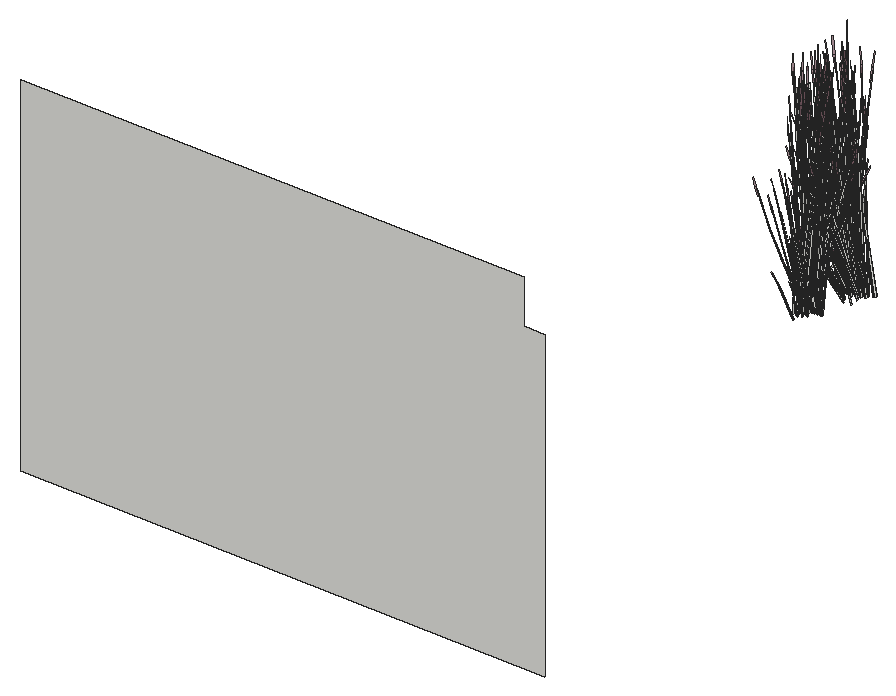
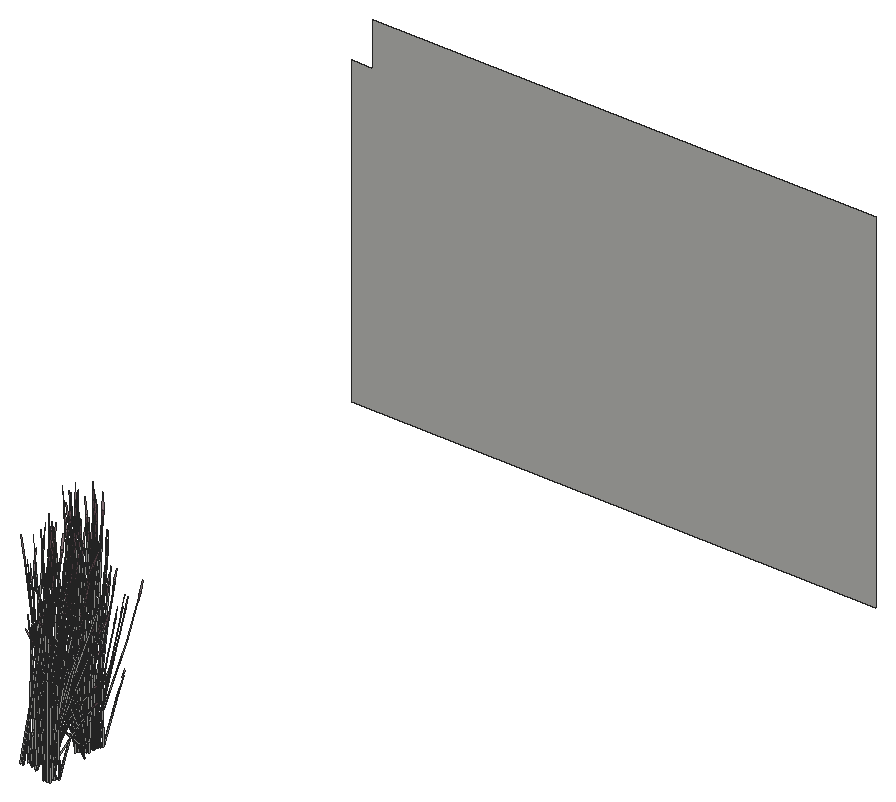
# SketchUp Ruby script. Lengths in inches.
U = 1.inch
M = Sketchup.active_model
def pt(a) = Geom::Point3d.new(a.map { |v| v * U })
def face(e, loops, mat)
  f = e.add_face(loops[0].map { |a| pt(a) })
  loops[1..].each { |l| e.add_face(l.map { |a| pt(a) }).erase! }
  f.material = f.back_material = mat if mat
  f
end
# faces: each face lists its corners as indices into pts; further lists are holes
def faces(e, pts, list, mat = nil) = list.each { |f| face(e, (f[0].is_a?(Array) ? f : [f]).map { |l| l.map { |i| pts[i] } }, mat) }
# xy, xz, yz: faces in a plane at the given z, y or x. An outline is a flat list of corners, or four numbers for a rectangle; further outlines are holes
def ring(l) = l.size == 4 ? [[l[0], l[1]], [l[2], l[1]], [l[2], l[3]], [l[0], l[3]]] : l.each_slice(2).to_a
def flat(e, list, mat, &to3) = list.each { |f| face(e, (f[0].is_a?(Array) ? f : [f]).map { |l| ring(l).map { |u, v| to3.(u, v) } }, mat) }
def xy(e, z, list, mat = nil) = flat(e, list, mat) { |x, y| [x, y, z] }
def xz(e, y, list, mat = nil) = flat(e, list, mat) { |x, z| [x, y, z] }
def yz(e, x, list, mat = nil) = flat(e, list, mat) { |y, z| [x, y, z] }
def lines(e, pts, list) = list.each { |a, b| e.add_line(pt(pts[a]), pt(pts[b])) }
# prism: a flat outline (further loops are holes) pulled along v
def prism(e, loops, v, mat = nil)
  f = face(e, loops, mat); d = Geom::Vector3d.new(v.map { |x| x * U })
  f.pushpull(f.normal.samedirection?(d) ? d.length : -d.length)
end
def box(e, o, s, mat = nil) = prism(e, [[o, [o[0] + s[0], o[1], o[2]], [o[0] + s[0], o[1] + s[1], o[2]], [o[0], o[1] + s[1], o[2]]]], [0, 0, s[2]], mat)
def at(x, y, z, deg = 0) = Geom::Transformation.translation(pt([x, y, z])) * Geom::Transformation.rotation(ORIGIN, Z_AXIS, deg.degrees)
def axes(o, x, y, z) = Geom::Transformation.new([*x, 0, *y, 0, *z, 0, *pt(o).to_a, 1])
def part(name) = M.definitions.add(name)
# library, detail: a bought-in or finely detailed component or shape, given as its bounding box
def library(name, o, s) = part(name).tap { |d| box(d.entities, o, s) }
def detail(e, o, s) = box(e.add_group.entities, o, s)
def put(e, d, t, mat = nil) = e.add_instance(d, t).tap { |i| i.material = mat if mat }
def group(e, t, mat = nil) = e.add_group.tap { |g| g.transformation = t; g.material = mat if mat }.entities
root = M.entities
M.materials.add("LightPink_Translucent").color = [144, 107, 117]
M.materials["LightPink_Translucent"].alpha = 0.75
c1 = part("blade")
p = [[2.15,0.21,22],[0,0.17,0],[0.09,0.45,0],[2.18,0.31,22],[2.29,0.31,22],[0.38,0.45,0],
  [2.48,0.24,33],[2.49,0.24,33],[2.48,0.22,33]]
faces(c1.entities,p,[[0,1,2,3],[4,5,2,3],[6,3,4,7],[8,0,3,6]])
c2 = part("seeds")
p = [[0.3,-0.1,1.38],[-0.01,-0.03,1.59],[-0.01,-0.03,0.03],[0.14,-0.07,-0.07],[0.29,-0.03,3],[0.15,0.01,3.11]]
faces(c2.entities,p,[[0,1,2,3],[1,0,4,5]],"LightPink_Translucent")
c3 = part("blade with seeds")
put(c3.entities,c1,at(0,0,0))
put(c3.entities,c2,axes([2.4,0.25,30.99],[1.5799,-0.05474,1.17369],[-0.12525,1.92788,0.29478],[-0.07173,-0.02425,1.56792]))
xz(root,279,[[198,0,342,0,342,84,336,84,336,96,198,96]])
put(root,c3,axes([289.94,432.61,2.59],[-0.25429,0.13207,1.43002],[-0.76157,-0.23115,-0.30754],[0.14117,-0.28747,0.61141]))
put(root,c3,axes([288.78,433.07,4.98],[-0.42698,-0.53052,-0.71045],[0.87893,-0.29566,0.08574],[-0.09984,-0.25633,1.00501]))
put(root,c3,axes([288.04,431.89,1.49],[-0.15005,0.02351,1.76342],[-0.82981,-0.26461,-0.26939],[0.01392,-0.22072,0.30037]))
put(root,c3,axes([290.55,433.59,4.98],[0.02328,-0.60353,-0.71045],[0.98022,0.04053,0.08574],[0.10344,-0.25568,1.00501]))
put(root,c3,axes([288.86,432.62,4.53],[0.2697,-0.50175,-0.35414],[0.78684,0.14635,0.4572],[-0.07215,-0.20201,0.87481]))
put(root,c3,axes([291.73,432.18,4.71],[-0.09085,0.04984,1.77383],[-0.89014,-0.16814,-0.16761],[-0.03222,-0.21748,0.31391]))
put(root,c3,axes([289,431.56,2.77],[0.11476,0.38047,1.1486],[-0.63664,-0.21072,0.84392],[0.06851,-0.19481,0.25299]))
put(root,c3,axes([290.36,433.39,4.68],[-0.64041,-0.4384,-0.51099],[0.67652,-0.38394,-0.3958],[0.09744,-0.22274,0.97773]))
put(root,c3,axes([288.95,432.74,4.73],[0.88151,0.17057,0.48003],[-0.30143,0.56078,0.3958],[-0.05297,-0.22053,0.9933]))
put(root,c3,axes([291.03,433.62,5.03],[-0.98321,-0.03233,-0.1216],[0.02687,-0.61208,-0.67495],[0.0683,-0.23574,1.02557]))
put(root,c3,axes([289.1875,432.69,4.73],[0.6592,-0.22175,0.0643],[0.32265,0.40436,0.50621],[-0.06366,-0.17825,0.77189]))
put(root,c3,axes([288.94,433.15,5.05],[-0.2697,0.50175,0.35414],[-0.78684,-0.14635,-0.4572],[-0.07215,-0.20201,0.87481]))
put(root,c3,axes([290.64,433.71,5.05],[-0.60531,0.34352,0.35414],[-0.573,-0.39225,-0.4572],[0.08718,-0.19929,0.87481]))
put(root,c3,axes([286.66,433.14,2.375],[-0.55932,-0.6538,0],[0.93577,-0.36461,-0.51607],[0.21313,-0.08304,1.63711]))
put(root,c3,axes([287.42,433.04,2.02],[0.83726,-0.32623,-0.49651],[0.50045,0.58498,0],[0.19069,-0.0743,1.57504]))
put(root,c3,axes([287.36,435.24,2.21],[0.43405,-0.58792,-0.44739],[0.90188,0.28295,0.21531],[0,-0.13553,1.43643]))
put(root,c3,axes([287.76,434.94,2.67],[-0.10425,-0.7445,-0.29095],[1.08575,-0.04502,-0.50002],[0.19119,-0.09917,1.59708]))
put(root,c3,axes([287.61,433.3,2.03],[0.83462,0.16144,-0.30978],[-0.21015,0.56852,0.30978],[0.16826,-0.06556,1.38974]))
put(root,c3,axes([287.9,435.53,2.43],[1.00799,0.31623,0.24065],[-0.48511,0.65709,0.50002],[0,-0.15147,1.60543]))
put(root,c3,axes([287.57,435.09,2.72],[-0.97146,0.04028,0.44739],[-0.08785,-0.66859,-0.21531],[0.17391,-0.06776,1.43643]))
put(root,c3,axes([287.54,435.33,2.36],[0.38895,0.72959,0.45755],[-1.11135,0.2537,0.17955],[0.01358,-0.13406,1.58856]))
put(root,c3,axes([287.34,435.9,2.72],[-0.43405,0.58792,0.44739],[-0.90188,-0.28295,-0.21531],[0,-0.13553,1.43643]))
put(root,c3,axes([288.9375,435.39,2.21],[0,-0.75495,0],[1.11865,0,0],[0,0,1.79456]))
put(root,c3,axes([290.29,433.65,2.48],[-0.83726,-0.32623,0.49651],[0.50045,-0.58498,0],[0.19069,0.0743,1.57504]))
put(root,c3,axes([288.41,434.91,2.36],[-0.74176,0.59212,0.45755],[-0.88124,-0.52269,0.17955],[0.17882,-0.05909,1.58856]))
put(root,c3,axes([289.22,435.97,2.3],[-0.83213,-0.56158,-0.06131],[0.83263,-0.56193,0],[-0.02906,-0.01961,1.75571]))
put(root,c3,axes([287.12,433.9375,2.47],[-0.25843,0.64844,0.17642],[-0.9457,-0.1835,0.35086],[0.16336,-0.00316,1.60407]))
put(root,c3,axes([289.09,434.66,2.62],[0.17258,-0.58229,0.1448],[0.84319,0.10108,-0.41347],[0.15345,0.05979,1.26744]))
put(root,c3,axes([288.73,434.8125,2.72],[-0.53742,-0.54764,0.44739],[0.81403,-0.38564,-0.21531],[0.17391,0.06776,1.43643]))
put(root,c3,axes([287.03,437.28,2.47],[0.96132,-0.17317,0.17642],[0.23737,0.64447,0.35086],[-0.08574,-0.0939,1.60407]))
put(root,c3,axes([289.7,435.56,2.21],[1.00089,0,0],[0,0.67548,0],[0,0,1.78407]))
put(root,c3,axes([289.98,433.97,2.47],[-0.96132,0.17317,0.17642],[-0.23737,-0.64447,0.35086],[0.08574,0.0939,1.60407]))
put(root,c3,axes([289.375,435.21,2.38],[-1.13071,-0.13747,0.49198],[0.23011,-0.77639,0.19306],[0.16524,0.07497,1.70813]))
put(root,c3,axes([288.47,437.13,2.2],[-0.29189,-0.56252,0],[0.83351,-0.19699,0],[0,0,1.54371]))
put(root,c3,axes([289.5625,437.05,2.18],[0.93921,-0.22138,-0.19198],[0.33003,0.6377,0.00008],[0.10367,-0.02447,1.73897]))
put(root,c3,axes([289.89,437.32,2.47],[0.25843,-0.64844,0.17642],[0.9457,0.1835,0.35086],[-0.16336,0.00316,1.60407]))
put(root,c3,axes([289.67,435.85,2.21],[0.62448,0.42144,0],[-0.62448,0.42144,0],[0,0,1.69266]))
put(root,c3,axes([291.37,435.66,2.47],[-0.70288,-0.47526,0.17642],[0.70832,-0.46097,0.35086],[-0.07763,0.09706,1.60407]))
put(root,c3,axes([288.27,437.39,2.2],[-0.90188,-0.29293,0],[0.43405,-0.60866,0],[0,0,1.62707]))
put(root,c3,axes([289.67,435.36,2.72],[0.43405,-0.58792,0.44739],[0.90188,0.28295,-0.21531],[0,0.13553,1.43643]))
put(root,c3,axes([289.5,435.69,2.29],[0,0.75458,-0.05637],[-1.11865,0,0],[0,0.02371,1.79368]))
put(root,c3,axes([291.94,435.68,2.48],[0,-0.65246,0.49651],[1.00089,0,0],[0,0.1486,1.57504]))
put(root,c3,axes([289.4375,436.17,2.72],[0.97146,-0.04028,0.44739],[0.08785,0.66859,-0.21531],[-0.17391,0.06776,1.43643]))
put(root,c3,axes([290.04,435.49,2.62],[0.83351,-0.19028,0.1448],[0.29189,0.54335,-0.41347],[0,0.11958,1.26744]))
put(root,c3,axes([289.29,437.4,2.2],[0.90188,0.29293,0],[-0.43405,0.60866,0],[0,0,1.74954]))
put(root,c3,axes([289.45,436.46,2.62],[0.66093,0.39201,0.1448],[-0.5513,0.44227,-0.41347],[-0.15345,0.05979,1.26744]))
put(root,c3,axes([290.16,437.67,2.48],[0.83726,-0.32623,0.49651],[0.50045,0.58498,0],[-0.19069,0.0743,1.57504]))
put(root,c3,axes([288.96,437.15,2.29],[0.38895,0.74956,-0.06012],[-1.11135,0.26265,0],[0.01358,0.02618,1.72173]))
put(root,c3,axes([292.18,436.17,2.2],[-1.1181,-0.00522,-0.04976],[0,-0.72922,0.49943],[-0.03514,0.166,1.58352]))
put(root,c3,axes([289.76,435.53,2.67],[1.00749,0.31132,-0.29095],[-0.48511,0.65709,-0.50002],[0.03166,0.16133,1.59708]))
put(root,c3,axes([292.51,444.75,3.875],[0.2045,0.20949,1.71376],[-0.94495,0.17636,0.13857],[-0.21357,-0.32887,0.73262]))
put(root,c3,axes([291.94,436.27,2.03],[-0.62448,0.40708,-0.30978],[-0.62448,-0.40708,0.30978],[0,0.13112,1.38974]))
put(root,c3,axes([289.65,436.02,2.21],[-0.43405,0.58792,-0.44739],[-0.90188,-0.28295,0.21531],[0,0.13553,1.43643]))
put(root,c3,axes([294.07,443.36,4.72],[-0.13683,-0.09148,1.74944],[-0.91315,0.058,-0.27667],[-0.14574,-0.2188,0.14031]))
put(root,c3,axes([295.02,444.9,4.98],[-0.42698,-0.53052,-0.71045],[0.87893,-0.29566,0.08574],[-0.09984,-0.25633,1.00501]))
put(root,c3,axes([292.25,444.19,2.59],[-0.05417,0.21344,1.43002],[-0.79196,0.17867,-0.30754],[-0.18512,-0.27588,0.61141]))
put(root,c3,axes([289.41,437.9,5.05],[-0.13817,-0.52554,0.35414],[0.78985,-0.13877,-0.4572],[0.21215,0.1506,0.87481]))
put(root,c3,axes([289.67,437.71,2.33],[1.11998,0.21207,0.30756],[-0.2802,0.75803,-0.36492],[-0.18537,0.09487,1.64885]))
put(root,c3,axes([292.375,436.29,2.02],[0,0.65246,-0.49651],[-1.00089,0,0],[0,0.1486,1.57504]))
put(root,c3,axes([294.7,444.8,4.68],[-0.87941,-0.16356,-0.51099],[0.30143,-0.56078,-0.3958],[-0.08064,-0.22578,0.97773]))
put(root,c3,axes([293.13,443.06,4.71],[-0.01669,0.07821,1.77383],[-0.82314,0.28383,-0.16761],[-0.24223,-0.14508,0.31391]))
put(root,c3,axes([290.35,438.12,2.375],[0.55932,0.6538,0],[-0.93577,0.36461,-0.51607],[-0.21313,0.08304,1.63711]))
put(root,c3,axes([290.16,436.2,2.09],[0.32803,0.59738,-0.69212],[-0.94492,0.21515,-0.18165],[0.03626,0.20229,1.52773]))
put(root,c3,axes([292.95,444.45,5.09],[0.99656,-0.1677,0.53763],[0.17295,0.65785,0.4433],[-0.23438,-0.19388,1.11249]))
put(root,c3,axes([287.52,437.99,5.05],[0.2697,-0.50175,0.35414],[0.78684,0.14635,-0.4572],[0.07215,0.20201,0.87481]))
put(root,c3,axes([295.46,444.77,5.03],[-0.87543,0.30377,-0.1216],[-0.4302,-0.53915,-0.67495],[-0.1155,-0.2272,1.02557]))
put(root,c3,axes([291.97,443.85,2.77],[0.46666,0.22709,1.1486],[-0.67962,0.13651,0.84392],[-0.14541,-0.17452,0.25299]))
put(root,c3,axes([293.1,445.05,4.98],[-0.76283,-0.31537,-0.71045],[0.54213,-0.55263,0.08574],[-0.27638,-0.1883,1.00501]))
put(root,c3,axes([292.84,444.64,4.53],[-0.13817,-0.52554,-0.35414],[0.78985,-0.13877,0.4572],[-0.21215,-0.1506,0.87481]))
put(root,c3,axes([289.53,438.38,4.73],[-0.4066,0.41448,0.0643],[-0.57901,-0.24131,0.50621],[0.18719,0.13288,0.77189]))
put(root,c3,axes([288.57,439.78,5.65],[0.61821,-0.37431,-0.06488],[0.56645,0.40995,-0.29416],[0.03988,0.11616,0.97024]))
put(root,c3,axes([289.7,438.27,4.73],[-0.88979,0.14973,0.48003],[-0.15442,-0.58737,0.3958],[0.20926,0.17311,0.9933]))
put(root,c3,axes([293.18,444.59,4.73],[0.4066,-0.41448,0.0643],[0.57901,0.24131,0.50621],[-0.18719,-0.13288,0.77189]))
put(root,c3,axes([291.6,444.53,1.49],[-0.08666,0.08595,1.76342],[-0.87574,0.18531,-0.26939],[-0.21156,-0.16858,0.30037]))
put(root,c3,axes([293.05,446.89,2.1],[-0.36739,-0.66907,-0.69835],[1.05831,-0.24096,-0.18329],[-0.04061,-0.22656,1.54149]))
put(root,c3,axes([287.27,438.44,4.73],[-0.6592,0.22175,0.0643],[-0.32265,-0.40436,0.50621],[0.06366,0.17825,0.77189]))
put(root,c3,axes([287.25,438.2,5.03],[0.87543,-0.30377,-0.1216],[0.4302,0.53915,-0.67495],[0.1155,0.2272,1.02557]))
put(root,c3,axes([287.51,438.4,5.0625],[-0.88151,-0.17057,0.53283],[0.30143,-0.56078,0.43934],[0.05297,0.22053,1.10256]))
put(root,c3,axes([292.74,445.07,4.68],[-0.88277,0.1551,-0.51099],[-0.15442,-0.58737,-0.3958],[-0.23711,-0.16832,0.97773]))
put(root,c3,axes([293.36,444.54,5.43],[-0.59706,0.6255,-0.13619],[-0.86465,-0.36036,-0.75594],[-0.30056,-0.17672,1.14864]))
put(root,c3,axes([287.41,438.32,1.49],[0.14478,-0.0355,1.76342],[0.8709,0.19542,-0.26939],[0.02547,0.22025,0.30037]))
put(root,c3,axes([294.13,444.18,2.13],[-0.61821,0.37431,-0.03893],[-0.56645,-0.40995,-0.17649],[-0.03988,-0.11616,0.58215]))
put(root,c3,axes([288,438.17,4.68],[0.87941,0.16356,-0.51099],[-0.30143,0.56078,-0.3958],[0.08064,0.22578,0.97773]))
put(root,c3,axes([288.5,437.02,3.875],[-0.2045,-0.20949,1.71376],[0.94495,-0.17636,0.13857],[0.21357,0.32887,0.73262]))
put(root,c3,axes([287.6,438.52,4.53],[-0.2697,0.50175,-0.35414],[-0.78684,-0.14635,0.4572],[0.07215,0.20201,0.87481]))
put(root,c3,axes([294.93,448.62,3.33],[0.77308,0.2631,1.51261],[-0.75736,0.56681,0.59816],[-0.33924,-0.33594,1.26806]))
put(root,c3,axes([293.3,445.0625,5.05],[0.13817,0.52554,0.35414],[-0.78985,0.13877,-0.4572],[-0.21215,-0.1506,0.87481]))
put(root,c3,axes([290.88,446.8,2.02],[0,-0.65246,-0.49651],[1.00089,0,0],[0,-0.1486,1.57504]))
put(root,c3,axes([287.68,438.07,4.98],[0.42698,0.53052,-0.71045],[-0.87893,0.29566,0.08574],[0.09984,0.25633,1.00501]))
put(root,c3,axes([291.27,445.4,4.73],[0.04505,-0.49615,0.0643],[0.68022,0.0136,0.50621],[-0.26056,-0.05192,0.77189]))
put(root,c3,axes([287.05,439.41,4.72],[0.1134,0.10507,1.74944],[0.91515,0.04128,-0.27667],[0.09203,0.23172,0.14031]))
put(root,c3,axes([291.3125,446.82,2.03],[0.62448,-0.40708,-0.30978],[0.62448,0.40708,0.30978],[0,-0.13112,1.38974]))
put(root,c3,axes([291.06,444.86,2.13],[-0.25807,0.53277,-0.03893],[-0.79428,-0.16389,-0.17649],[-0.1206,-0.08714,0.58215]))
put(root,c3,axes([293.5,447.56,2.67],[-1.00749,-0.31132,-0.29095],[0.48511,-0.65709,-0.50002],[-0.03166,-0.16133,1.59708]))
put(root,c3,axes([290.63,447.3,2.375],[-1.11865,0,0],[0,-0.72922,-0.51607],[0,-0.16609,1.63711]))
put(root,c3,axes([288.49,449.68,2.59],[-0.25429,0.13207,1.43002],[-0.76157,-0.23115,-0.30754],[0.14117,-0.28747,0.61141]))
put(root,c3,axes([286.6,448.96,1.49],[-0.15005,0.02351,1.76342],[-0.82981,-0.26461,-0.26939],[0.01392,-0.22072,0.30037]))
put(root,c3,axes([291.5,447.1,2.33],[-0.83213,0.54855,0.30756],[-0.83263,-0.54278,-0.36492],[-0.02906,-0.15578,1.64885]))
put(root,c3,axes([289.11,450.66,4.98],[0.02328,-0.60353,-0.71045],[0.98022,0.04053,0.08574],[0.10344,-0.25568,1.00501]))
put(root,c3,axes([293.75,448.25,2.4375],[0.23711,-0.77313,-0.23429],[1.12425,0.13477,0.51271],[-0.19645,-0.10677,1.5644]))
put(root,c3,axes([290.48,449.71,4.72],[-0.00864,-0.12985,1.74944],[-0.72937,-0.3753,-0.27667],[0.11277,-0.2275,0.14031]))
put(root,c3,axes([287.41,449.6875,4.53],[0.2697,-0.50175,-0.35414],[0.78684,0.14635,0.4572],[-0.07215,-0.20201,0.87481]))
put(root,c3,axes([290.28,449.25,4.71],[-0.09085,0.04984,1.77383],[-0.89014,-0.16814,-0.16761],[-0.03222,-0.21748,0.31391]))
put(root,c3,axes([291.73,445.77,5.05],[0.50902,0.40851,0.35414],[-0.58122,0.38671,-0.4572],[-0.29531,-0.05884,0.87481]))
put(root,c3,axes([287.56,448.625,2.77],[0.11476,0.38047,1.1486],[-0.63664,-0.21072,0.84392],[0.06851,-0.19481,0.25299]))
put(root,c3,axes([291.3125,447.41,2.48],[0,0.65246,0.49651],[-1.00089,0,0],[0,-0.1486,1.57504]))
put(root,c3,axes([288.91,450.46,4.68],[-0.64041,-0.4384,-0.51099],[0.67652,-0.38394,-0.3958],[0.09744,-0.22274,0.97773]))
put(root,c3,axes([293.68,447.93,2.21],[-0.53742,-0.54764,-0.44739],[0.81403,-0.38564,0.21531],[-0.17391,-0.06776,1.43643]))
put(root,c3,axes([293.59,447.73,2.72],[-0.43405,0.58792,0.44739],[-0.90188,-0.28295,-0.21531],[0,-0.13553,1.43643]))
put(root,c3,axes([287.51,449.8,4.73],[0.88151,0.17057,0.48003],[-0.30143,0.56078,0.3958],[-0.05297,-0.22053,0.9933]))
put(root,c3,axes([289.58,450.6875,5.03],[-0.98321,-0.03233,-0.1216],[0.02687,-0.61208,-0.67495],[0.0683,-0.23574,1.02557]))
put(root,c3,axes([289.51,450.29,4.53],[0.60531,-0.34352,-0.35414],[0.573,0.39225,0.4572],[0.08718,-0.19929,0.87481]))
put(root,c3,axes([287.75,449.76,4.73],[0.6592,-0.22175,0.0643],[0.32265,0.40436,0.50621],[-0.06366,-0.17825,0.77189]))
put(root,c3,axes([293.19,448.14,2.06],[-0.9306,-0.10697,-0.62353],[0.19638,-0.65984,-0.16365],[-0.27771,-0.07995,1.37633]))
put(root,c3,axes([293.88,447.875,2.36],[1.13071,0.13747,0.45755],[-0.23011,0.77639,0.17955],[-0.16524,-0.07497,1.58856]))
put(root,c3,axes([292.2,449.15,2.03],[-0.21015,-0.56852,-0.30978],[0.83462,-0.16144,0.30978],[-0.16826,-0.06556,1.38974]))
put(root,c3,axes([293.28,449.12,2.47],[0.96132,-0.17317,0.17642],[0.23737,0.64447,0.35086],[-0.08574,-0.0939,1.60407]))
put(root,c3,axes([289.51,450.43,4.73],[0.63704,0.44518,0.48003],[-0.67652,0.38394,0.3958],[0.11751,-0.20886,0.9933]))
put(root,c3,axes([289.75,450.47,4.73],[0.73517,0.0304,0.0643],[-0.02016,0.45906,0.50621],[0.07693,-0.17585,0.77189]))
put(root,c3,axes([291.97,449.39,2.02],[-0.83726,-0.32623,-0.49651],[0.50045,-0.58498,0],[-0.19069,-0.0743,1.57504]))
put(root,c3,axes([289.2,450.78,5.05],[-0.60531,0.34352,0.35414],[-0.573,-0.39225,-0.4572],[0.08718,-0.19929,0.87481]))
put(root,c3,axes([294.25,448.24,2.67],[-0.90324,0.43318,-0.29095],[-0.60064,-0.61207,-0.50002],[-0.22285,-0.06216,1.59708]))
put(root,c3,axes([285.21,450.21,2.375],[-0.55932,-0.6538,0],[0.93577,-0.36461,-0.51607],[0.21313,-0.08304,1.63711]))
put(root,c3,axes([294.16,448.43,2.62],[-0.17258,0.58229,0.1448],[-0.84319,-0.10108,-0.41347],[-0.15345,-0.05979,1.26744]))
put(root,c3,axes([290.89,446.92,5.05],[0.74348,0.18202,0.35414],[-0.21685,0.53102,-0.4572],[-0.29933,0.04869,0.87481]))
put(root,c3,axes([285.97,450.1,2.02],[0.83726,-0.32623,-0.49651],[0.50045,0.58498,0],[0.19069,-0.0743,1.57504]))
put(root,c3,axes([286.97,451.44,2.06],[0.60257,-0.49041,-0.62353],[0.74854,0.44469,-0.16365],[0.24146,-0.12234,1.37633]))
put(root,c3,axes([295.26,448.4375,2.46],[-0.87356,-0.52515,-0.25192],[0.73507,-0.5897,0.5513],[-0.23523,0.06143,1.68216]))
put(root,c3,axes([292.96,449.44,2.48],[0.83726,0.32623,0.49651],[-0.50045,0.58498,0],[-0.19069,-0.0743,1.57504]))
put(root,c3,axes([285.92,452.3,2.21],[0.43405,-0.58792,-0.44739],[0.90188,0.28295,0.21531],[0,-0.13553,1.43643]))
put(root,c3,axes([286.3125,452.01,2.67],[-0.10425,-0.7445,-0.29095],[1.08575,-0.04502,-0.50002],[0.19119,-0.09917,1.59708]))
put(root,c3,axes([292.48,449.79,2.375],[-0.55932,0.6538,0],[-0.93577,-0.36461,-0.51607],[-0.21313,-0.08304,1.63711]))
put(root,c3,axes([290.25,451.84,5.05],[-0.77872,0.09325,0.35414],[-0.20563,-0.53305,-0.4572],[0.22316,-0.14318,0.87481]))
put(root,c3,axes([294.82,448.33,2.21],[-0.97146,0.04028,-0.44739],[-0.08785,-0.66859,0.21531],[-0.17391,0.06776,1.43643]))
put(root,c3,axes([286.17,450.36,2.03],[0.83462,0.16144,-0.30978],[-0.21015,0.56852,0.30978],[0.16826,-0.06556,1.38974]))
put(root,c3,axes([295.9,449.88,2.19],[-0.55235,-0.65609,-0.05142],[0.93577,-0.36461,0.51607],[-0.23059,0.06247,1.6363]))
put(root,c3,axes([286.46,452.59,2.43],[1.00799,0.31623,0.24065],[-0.48511,0.65709,0.50002],[0,-0.15147,1.60543]))
put(root,c3,axes([295.64,449.79,2.03],[-0.83462,-0.16144,-0.30978],[0.21015,-0.56852,0.30978],[-0.16826,0.06556,1.38974]))
put(root,c3,axes([291.02,448.19,5.05],[0.77872,-0.09325,0.35414],[0.20563,0.53305,-0.4572],[-0.22316,0.14318,0.87481]))
put(root,c3,axes([286.13,452.15,2.72],[-0.97146,0.04028,0.44739],[-0.08785,-0.66859,-0.21531],[0.17391,-0.06776,1.43643]))
put(root,c3,axes([295.5,448.15,2.67],[0.10425,0.7445,-0.29095],[-1.08575,0.04502,-0.50002],[-0.19119,0.09917,1.59708]))
put(root,c3,axes([286.1,452.4,2.36],[0.38895,0.72959,0.45755],[-1.11135,0.2537,0.17955],[0.01358,-0.13406,1.58856]))
put(root,c3,axes([287.5,452.46,2.21],[0,-0.75495,0],[1.11865,0,0],[0,0,1.79456]))
put(root,c3,axes([288.85,450.71,2.48],[-0.83726,-0.32623,0.49651],[0.50045,-0.58498,0],[0.19069,0.0743,1.57504]))
